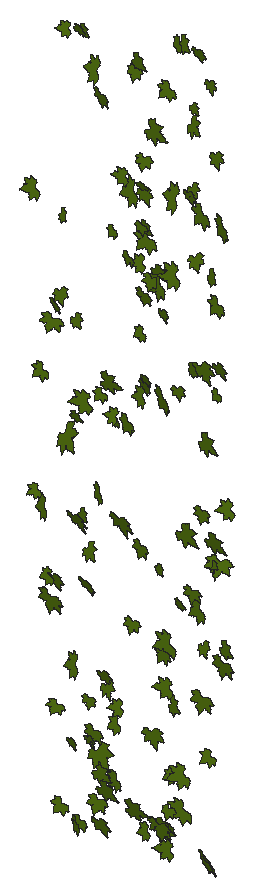
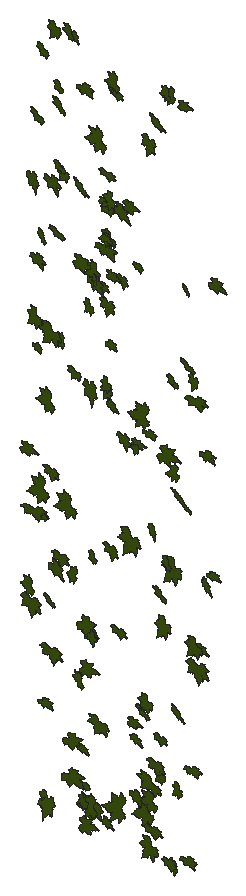
# SketchUp Ruby script. Lengths in inches.
U = 1.inch
M = Sketchup.active_model
def pt(a) = Geom::Point3d.new(a.map { |v| v * U })
def face(e, loops, mat)
  f = e.add_face(loops[0].map { |a| pt(a) })
  loops[1..].each { |l| e.add_face(l.map { |a| pt(a) }).erase! }
  f.material = f.back_material = mat if mat
  f
end
# faces: each face lists its corners as indices into pts; further lists are holes
def faces(e, pts, list, mat = nil) = list.each { |f| face(e, (f[0].is_a?(Array) ? f : [f]).map { |l| l.map { |i| pts[i] } }, mat) }
# xy, xz, yz: faces in a plane at the given z, y or x. An outline is a flat list of corners, or four numbers for a rectangle; further outlines are holes
def ring(l) = l.size == 4 ? [[l[0], l[1]], [l[2], l[1]], [l[2], l[3]], [l[0], l[3]]] : l.each_slice(2).to_a
def flat(e, list, mat, &to3) = list.each { |f| face(e, (f[0].is_a?(Array) ? f : [f]).map { |l| ring(l).map { |u, v| to3.(u, v) } }, mat) }
def xy(e, z, list, mat = nil) = flat(e, list, mat) { |x, y| [x, y, z] }
def xz(e, y, list, mat = nil) = flat(e, list, mat) { |x, z| [x, y, z] }
def yz(e, x, list, mat = nil) = flat(e, list, mat) { |y, z| [x, y, z] }
def lines(e, pts, list) = list.each { |a, b| e.add_line(pt(pts[a]), pt(pts[b])) }
# prism: a flat outline (further loops are holes) pulled along v
def prism(e, loops, v, mat = nil)
  f = face(e, loops, mat); d = Geom::Vector3d.new(v.map { |x| x * U })
  f.pushpull(f.normal.samedirection?(d) ? d.length : -d.length)
end
def box(e, o, s, mat = nil) = prism(e, [[o, [o[0] + s[0], o[1], o[2]], [o[0] + s[0], o[1] + s[1], o[2]], [o[0], o[1] + s[1], o[2]]]], [0, 0, s[2]], mat)
def at(x, y, z, deg = 0) = Geom::Transformation.translation(pt([x, y, z])) * Geom::Transformation.rotation(ORIGIN, Z_AXIS, deg.degrees)
def axes(o, x, y, z) = Geom::Transformation.new([*x, 0, *y, 0, *z, 0, *pt(o).to_a, 1])
def part(name) = M.definitions.add(name)
# library, detail: a bought-in or finely detailed component or shape, given as its bounding box
def library(name, o, s) = part(name).tap { |d| box(d.entities, o, s) }
def detail(e, o, s) = box(e.add_group.entities, o, s)
def put(e, d, t, mat = nil) = e.add_instance(d, t).tap { |i| i.material = mat if mat }
def group(e, t, mat = nil) = e.add_group.tap { |g| g.transformation = t; g.material = mat if mat }.entities
root = M.entities
M.materials.add("[Vegetation Blur 03]").color = [83, 114, 18]
c1 = part("ivy")
xy(c1.entities,0,[[0.782,0,0.786,0,0.787,0.005,0.789,0.009,0.821,0.072,0.875,0.147,1.001,0.272,1.073,0.331,1.137,0.363,1.178,0.379,1.223,0.384,1.272,0.383,1.311,0.374,1.36,0.355,1.399,0.334,1.491,0.285,1.541,0.244,1.583,0.199,1.617,0.15,1.64,0.128,1.662,0.115,1.717,0.105,1.745,0.093,1.784,0.054,1.819,0.057,1.854,0.064,1.882,0.075,1.896,0.074,1.91,0.071,1.937,0.063,1.964,0.053,1.99,0.038,2.016,0.015,2.034,0.002,2.04,0,2.038,0.003,2.036,0.007,2.033,0.038,2.036,0.068,2.045,0.1,2.055,0.116,2.064,0.123,2.077,0.129,2.088,0.129,2.106,0.132,2.118,0.13,2.179,0.132,2.207,0.133,2.225,0.133,2.242,0.138,2.22,0.162,2.207,0.186,2.206,0.213,2.212,0.236,2.228,0.262,2.247,0.274,2.298,0.283,2.355,0.294,2.37,0.296,2.376,0.295,2.377,0.3,2.377,0.303,2.385,0.329,2.411,0.37,2.426,0.392,2.449,0.407,2.511,0.426,2.561,0.444,2.619,0.466,2.589,0.469,2.561,0.476,2.501,0.5,2.449,0.516,2.424,0.523,2.401,0.535,2.377,0.556,2.372,0.568,2.36,0.575,2.268,0.586,2.225,0.592,2.207,0.599,2.194,0.61,2.143,0.65,2.13,0.664,2.122,0.682,2.123,0.7,2.13,0.719,2.148,0.75,2.17,0.781,2.195,0.807,2.221,0.828,2.284,0.874,2.291,0.88,2.288,0.887,2.276,0.9,2.267,0.916,2.265,0.933,2.273,0.967,2.292,1.002,2.313,1.03,2.334,1.054,2.348,1.067,2.358,1.074,2.363,1.076,2.362,1.081,2.35,1.094,2.347,1.11,2.35,1.143,2.359,1.18,2.385,1.254,2.415,1.324,2.448,1.393,2.45,1.4,2.446,1.398,2.44,1.394,2.427,1.383,2.402,1.36,2.376,1.339,2.345,1.324,2.305,1.309,2.282,1.303,2.273,1.306,2.245,1.294,2.212,1.287,2.187,1.291,2.163,1.301,2.142,1.316,2.134,1.327,2.124,1.325,2.09,1.292,2.053,1.259,2.014,1.234,1.973,1.215,1.954,1.21,1.931,1.208,1.909,1.212,1.893,1.22,1.879,1.233,1.872,1.248,1.867,1.281,1.864,1.319,1.821,1.258,1.773,1.197,1.726,1.141,1.698,1.121,1.679,1.116,1.666,1.117,1.647,1.122,1.632,1.129,1.62,1.141,1.617,1.154,1.617,1.219,1.621,1.254,1.623,1.268,1.623,1.281,1.618,1.314,1.606,1.346,1.603,1.375,1.607,1.403,1.603,1.467,1.599,1.499,1.605,1.525,1.614,1.552,1.629,1.577,1.635,1.589,1.629,1.587,1.618,1.582,1.596,1.566,1.581,1.556,1.568,1.552,1.557,1.55,1.545,1.553,1.531,1.562,1.522,1.572,1.504,1.591,1.486,1.611,1.474,1.631,1.457,1.666,1.455,1.684,1.457,1.698,1.452,1.715,1.444,1.728,1.424,1.754,1.419,1.772,1.423,1.786,1.434,1.819,1.444,1.848,1.446,1.855,1.44,1.861,1.43,1.867,1.386,1.904,1.349,1.948,1.326,1.973,1.31,1.995,1.288,2.048,1.284,2.153,1.287,2.254,1.284,2.255,1.282,2.253,1.278,2.247,1.274,2.237,1.266,2.216,1.226,2.125,1.208,2.076,1.184,2.033,1.155,1.984,1.135,1.942,1.111,1.899,1.083,1.861,1.053,1.85,1.059,1.83,1.061,1.809,1.056,1.79,1.049,1.767,1.04,1.749,1.018,1.733,0.994,1.726,0.942,1.734,0.95,1.6875,0.944,1.645,0.932,1.608,0.911,1.585,0.881,1.58,0.854,1.582,0.828,1.588,0.785,1.618,0.773,1.625,0.775,1.614,0.779,1.598,0.796,1.502,0.818,1.402,0.861,1.283,0.882,1.224,0.894,1.174,0.892,1.148,0.886,1.123,0.881,1.107,0.872,1.099,0.849,1.094,0.818,1.092,0.789,1.098,0.762,1.107,0.753,1.113,0.721,1.139,0.698,1.163,0.678,1.194,0.665,1.224,0.628,1.28,0.612,1.312,0.606,1.327,0.606,1.314,0.599,1.282,0.594,1.267,0.581,1.256,0.544,1.245,0.512,1.244,0.473,1.249,0.444,1.256,0.382,1.288,0.339,1.306,0.324,1.316,0.317,1.324,0.309,1.326,0.27,1.314,0.227,1.313,0.185,1.3125,0.152,1.317,0.122,1.328,0.092,1.345,0.073,1.353,0.079,1.338,0.092,1.308,0.117,1.249,0.13,1.215,0.139,1.164,0.147,1.148,0.157,1.136,0.163,1.122,0.174,1.086,0.177,1.067,0.182,1.054,0.186,1.043,0.191,1.038,0.211,1.028,0.237,1.005,0.25,0.974,0.253,0.96,0.25,0.944,0.242,0.914,0.243,0.906,0.249,0.902,0.26,0.894,0.289,0.88,0.307,0.873,0.322,0.862,0.364,0.799,0.403,0.738,0.431,0.709,0.439,0.691,0.441,0.678,0.4375,0.66,0.428,0.645,0.394,0.623,0.303,0.594,0.255,0.581,0.214,0.577,0.179,0.573,0.173,0.568,0.175,0.561,0.167,0.55,0.141,0.523,0.113,0.503,0.077,0.49,0.045,0.486,0.026,0.485,0.019,0.486,0.011,0.483,0,0.471,0.014,0.467,0.044,0.455,0.058,0.447,0.07,0.438,0.097,0.411,0.125,0.394,0.158,0.377,0.174,0.366,0.182,0.359,0.185,0.361,0.242,0.331,0.253,0.316,0.258,0.303,0.262,0.283,0.274,0.278,0.308,0.274,0.341,0.252,0.366,0.226,0.366,0.222,0.37,0.22,0.38,0.221,0.395,0.221,0.425,0.216,0.45,0.207,0.465,0.192,0.473,0.178,0.484,0.15,0.489,0.116,0.483,0.089,0.468,0.058,0.45,0.035,0.435,0.018,0.429,0.011,0.434,0.012,0.438,0.014,0.469,0.019,0.542,0.016,0.581,0.015,0.612,0.027,0.68,0.055,0.696,0.057,0.712,0.052,0.73,0.045,0.741,0.036,0.766,0.014]])
put(root,c1,axes([10.7,173.7,38.86],[0.22705,-0.11945,-0.35491],[-0.43835,-0.02,-0.18572],[-0.01818,-1.0093,0.04569]),"[Vegetation Blur 03]")
put(root,c1,axes([10.72,173.7,22.84],[0.22258,-0.06561,-0.19839],[-0.24493,-0.08915,-0.17839],[0.01076,-0.67235,0.04301]),"[Vegetation Blur 03]")
put(root,c1,axes([10.9375,173.7,29.33],[0.3254,-0.08509,-0.21734],[-0.269,-0.05049,-0.26515],[-0.01633,-0.86378,0.03691]),"[Vegetation Blur 03]")
put(root,c1,axes([11.23,173.7,22.41],[0.27571,-0.25978,-0.33675],[-0.40528,0.18997,-0.24407],[-0.14812,-1.00337,0.04098]),"[Vegetation Blur 03]")
put(root,c1,axes([11.59,173.7,18.67],[0.1748,-0.10036,-0.26156],[-0.32362,-0.01023,-0.14344],[-0.01895,-0.75115,0.0369]),"[Vegetation Blur 03]")
put(root,c1,axes([11.22,173.7,32.02],[0.48108,0.0091,-0.09014],[-0.10924,-0.11608,-0.39016],[0.0169,-1.00907,0.04407]),"[Vegetation Blur 03]")
put(root,c1,axes([10.97,173.7,17.55],[0.65346,-0.15996,-0.07236],[-0.08578,0.05992,-0.53686],[-0.0809,-1.3557,-0.01519]),"[Vegetation Blur 03]")
put(root,c1,axes([11.625,173.7,11.875],[0.36198,-0.00364,-0.10329],[-0.12566,-0.10485,-0.29275],[0.01516,-0.7821,0.03972]),"[Vegetation Blur 03]")
put(root,c1,axes([11.57,173.7,32.88],[0.3582,-0.18702,-0.03708],[-0.03384,0.10347,-0.29982],[-0.09581,-0.73577,-0.03274]),"[Vegetation Blur 03]")
put(root,c1,axes([11.21,173.7,18.26],[0.44883,-0.14962,0.17944],[0.22549,0.05754,-0.36812],[-0.05276,-1.02686,-0.04677]),"[Vegetation Blur 03]")
put(root,c1,axes([11.97,173.7,6.9],[0.37574,-0.07096,-0.15978],[-0.19839,-0.07956,-0.3052],[-0.01253,-0.86822,0.04103]),"[Vegetation Blur 03]")
put(root,c1,axes([11.74,173.7,33.23],[0.32579,-0.0019,0.20222],[0.24053,-0.19974,-0.25841],[-0.05947,-0.81825,0.06261]),"[Vegetation Blur 03]")
put(root,c1,axes([12.07,173.7,37.17],[0.07732,0.04701,0.24249],[0.28519,-0.19481,-0.05463],[-0.0864,-0.60099,0.03668]),"[Vegetation Blur 03]")
put(root,c1,axes([12.75,173.7,47.72],[0.09099,-0.0894,-0.27257],[-0.33609,-0.07013,-0.07111],[0.02177,-0.70885,0.04141]),"[Vegetation Blur 03]")
put(root,c1,axes([11.88,173.7,25.39],[0.26041,0.16269,0.49935],[0.59768,-0.40532,-0.18684],[-0.15294,-1.30696,0.1201]),"[Vegetation Blur 03]")
put(root,c1,axes([13.15,173.7,14.82],[0.25932,-0.29593,-0.35358],[-0.43934,0.11655,-0.22996],[-0.12392,-1.03246,0.07539]),"[Vegetation Blur 03]")
put(root,c1,axes([12.51,173.7,10.03],[0.27088,-0.15261,0.15464],[0.19269,-0.01614,-0.22733],[-0.06536,-0.68006,-0.0293]),"[Vegetation Blur 03]")
put(root,c1,axes([12.92,173.7,6.22],[0.37274,-0.27698,-0.10257],[-0.11734,0.09274,-0.32343],[-0.14192,-0.80413,-0.00197]),"[Vegetation Blur 03]")
put(root,c1,axes([12.75,173.7,26.97],[0.1451,-0.1312,0.25798],[0.3214,0.00081,-0.12034],[-0.02623,-0.71573,-0.04743]),"[Vegetation Blur 03]")
put(root,c1,axes([12.72,173.7,32.03],[0.20968,0.01131,0.23173],[0.28004,-0.12895,-0.16779],[-0.0472,-0.71481,0.03394]),"[Vegetation Blur 03]")
put(root,c1,axes([13.78,173.7,28.72],[0.17219,-0.03701,-0.43547],[-0.53302,-0.07752,-0.13935],[0.03036,-1.15115,0.02338]),"[Vegetation Blur 03]")
put(root,c1,axes([13.04,173.7,6.29],[0.37414,-0.10141,-0.07585],[-0.09511,-0.0243,-0.3074],[-0.04493,-0.79294,0.01912]),"[Vegetation Blur 03]")
put(root,c1,axes([12.45,173.7,21.96],[0.55336,-0.2755,0.17895],[0.23761,0.14136,-0.45516],[-0.0977,-1.21665,-0.0934]),"[Vegetation Blur 03]")
put(root,c1,axes([12.97,173.7,47.37],[0.16816,-0.15089,0.24654],[0.3088,-0.00002,-0.1403],[-0.03567,-0.71145,-0.05229]),"[Vegetation Blur 03]")
put(root,c1,axes([13.19,173.7,21.9],[0.13772,-0.02232,0.26418],[0.31478,-0.16115,-0.11144],[-0.07624,-0.70573,0.01709]),"[Vegetation Blur 03]")
put(root,c1,axes([13.25,173.7,47.37],[0.14289,-0.07488,0.25812],[0.31299,-0.09737,-0.11985],[-0.0582,-0.70749,-0.01082]),"[Vegetation Blur 03]")
put(root,c1,axes([13.14,173.7,18.76],[0.46892,-0.24319,0.11777],[0.16224,0.13537,-0.38629],[-0.09203,-1.00049,-0.08089]),"[Vegetation Blur 03]")
put(root,c1,axes([13.48,173.7,12.71],[0.35341,-0.05372,0.02619],[0.03014,-0.05475,-0.28854],[-0.02834,-0.72817,0.01976]),"[Vegetation Blur 03]")
put(root,c1,axes([13.51,173.7,10.5],[0.29444,-0.13699,0.14225],[0.1786,0.0132,-0.24425],[-0.05394,-0.70397,-0.03226]),"[Vegetation Blur 03]")
put(root,c1,axes([13.42,173.7,20.09],[0.20883,0.04815,0.31421],[0.37772,-0.20796,-0.1622],[-0.0781,-0.87697,0.05572]),"[Vegetation Blur 03]")
put(root,c1,axes([14.55,173.7,46.43],[0.1383,-0.27518,-0.42018],[-0.52123,0.14835,-0.12955],[-0.10615,-1.08693,0.0887]),"[Vegetation Blur 03]")
put(root,c1,axes([13.69,173.7,11.3],[0.4987,-0.12613,-0.04723],[-0.0598,-0.02572,-0.40975],[-0.05942,-1.03278,0.01597]),"[Vegetation Blur 03]")
put(root,c1,axes([14.34,173.7,24.12],[0.31941,-0.24553,-0.21108],[-0.24847,0.1507,-0.27802],[-0.13923,-0.8322,0.01193]),"[Vegetation Blur 03]")
put(root,c1,axes([13.91,173.7,7.7],[0.48615,-0.06506,-0.03255],[-0.04363,-0.12709,-0.39413],[-0.0262,-0.99568,0.05243]),"[Vegetation Blur 03]")
put(root,c1,axes([14.4,173.7,29.18],[0.29981,-0.06525,-0.13535],[-0.1686,-0.07812,-0.24283],[-0.00912,-0.70071,0.03968]),"[Vegetation Blur 03]")
put(root,c1,axes([14.13,173.7,44.84],[0.50217,-0.23211,-0.02067],[-0.01614,0.08923,-0.41886],[-0.11447,-1.03084,-0.03161]),"[Vegetation Blur 03]")
put(root,c1,axes([13.66,173.7,9.65],[0.43574,0.04341,0.40329],[0.4922,-0.17124,-0.35133],[-0.04861,-1.34487,0.05775]),"[Vegetation Blur 03]")
put(root,c1,axes([13.98,173.7,8.53],[0.18345,-0.01602,0.41607],[0.50825,-0.08298,-0.14976],[-0.04057,-1.11184,0.00518]),"[Vegetation Blur 03]")
put(root,c1,axes([13.875,173.7,6.36],[0.49317,-0.18476,0.20262],[0.2548,0.0498,-0.40595],[-0.06909,-1.1351,-0.05079]),"[Vegetation Blur 03]")
put(root,c1,axes([14.24,173.7,14.15],[0.36419,-0.14328,0.1768],[0.2225,0.04791,-0.29916],[-0.04769,-0.87068,-0.04556]),"[Vegetation Blur 03]")
put(root,c1,axes([14.2,173.7,7.85],[0.29611,-0.16504,0.41768],[0.51687,0.01316,-0.24325],[-0.03458,-1.21665,-0.05929]),"[Vegetation Blur 03]")
put(root,c1,axes([14.48,173.7,13.44],[0.29238,-0.00543,0.2431],[0.28843,-0.20948,-0.23179],[-0.07444,-0.83296,0.05671]),"[Vegetation Blur 03]")
put(root,c1,axes([15.62,173.7,28.375],[0.04403,-0.12753,-0.27738],[-0.34532,-0.03734,-0.03381],[0.01033,-0.70424,0.05202]),"[Vegetation Blur 03]")
put(root,c1,axes([15.09,173.7,37.94],[0.27643,-0.11245,-0.0959],[-0.1208,-0.01738,-0.22873],[-0.04691,-0.61786,0.02389]),"[Vegetation Blur 03]")
put(root,c1,axes([14.59,173.7,29.11],[0.08822,-0.12322,0.46198],[0.56917,0.00464,-0.0722],[-0.00698,-1.17889,-0.04857]),"[Vegetation Blur 03]")
put(root,c1,axes([15.27,173.7,9.4],[0.34978,-0.17504,-0.23097],[-0.28247,0.06704,-0.29293],[-0.08681,-0.92345,0.02252]),"[Vegetation Blur 03]")
put(root,c1,axes([15.43,173.7,12.375],[0.28202,-0.18926,-0.22565],[-0.28437,-0.00619,-0.23592],[-0.06351,-0.81269,0.05435]),"[Vegetation Blur 03]")
put(root,c1,axes([15.18,173.7,27.98],[0.28723,-0.15203,-0.02555],[-0.02588,0.0511,-0.24162],[-0.07595,-0.59236,-0.01429]),"[Vegetation Blur 03]")
put(root,c1,axes([15.79,173.7,13.22],[0.11929,-0.10597,-0.2818],[-0.34889,-0.06251,-0.09467],[0.01224,-0.74914,0.04776]),"[Vegetation Blur 03]")
put(root,c1,axes([16.11,173.7,41.16],[0.05825,-0.05857,-0.32384],[-0.39732,-0.0501,-0.04618],[0.02002,-0.82377,0.02584]),"[Vegetation Blur 03]")
put(root,c1,axes([14.96,173.7,22.8],[0.63866,-0.23189,0.12864],[0.16822,0.10928,-0.52532],[-0.09614,-1.34925,-0.06466]),"[Vegetation Blur 03]")
put(root,c1,axes([15.83,173.7,28.36],[0.44792,-0.20906,-0.13241],[-0.16237,0.03502,-0.37455],[-0.10139,-0.9797,0.01487]),"[Vegetation Blur 03]")
put(root,c1,axes([15.92,173.7,36.87],[0.35103,-0.1488,-0.07514],[-0.0909,0.03087,-0.29249],[-0.07377,-0.74614,0.00288]),"[Vegetation Blur 03]")
put(root,c1,axes([16.41,173.7,40.93],[0.36429,-0.26691,-0.39719],[-0.49048,0.09297,-0.30946],[-0.1145,-1.24751,0.06192]),"[Vegetation Blur 03]")
put(root,c1,axes([16,173.7,17.7],[0.40879,-0.06868,-0.00639],[-0.01176,-0.09983,-0.33231],[-0.0322,-0.83542,0.04024]),"[Vegetation Blur 03]")
put(root,c1,axes([16.21,173.7,46.72],[0.38042,-0.08348,0.02066],[0.01844,-0.12918,-0.30833],[-0.04412,-0.77385,0.04924]),"[Vegetation Blur 03]")
put(root,c1,axes([17.07,173.7,37.02],[0.14335,-0.13764,-0.29117],[-0.36286,-0.03379,-0.11648],[-0.00945,-0.79049,0.05568]),"[Vegetation Blur 03]")
put(root,c1,axes([17.05,173.7,30.09],[0.18991,-0.19032,-0.31472],[-0.38839,0.08836,-0.16451],[-0.08006,-0.88012,0.05154]),"[Vegetation Blur 03]")
put(root,c1,axes([16.05,173.7,7.26],[0.11966,-0.19885,0.48664],[0.60405,0.04067,-0.09632],[0.00062,-1.25082,-0.0805]),"[Vegetation Blur 03]")
put(root,c1,axes([16.91,173.7,33.25],[0.22039,-0.10268,-0.20891],[-0.2592,-0.01,-0.18136],[-0.02883,-0.69502,0.03347]),"[Vegetation Blur 03]")
put(root,c1,axes([16.34,173.7,46.71],[0.15082,-0.08194,0.36497],[0.44384,-0.11913,-0.12637],[-0.06768,-0.96384,-0.01541]),"[Vegetation Blur 03]")
put(root,c1,axes([16.52,173.7,21.99],[0.46442,-0.17928,-0.04706],[-0.05947,-0.00913,-0.38545],[-0.0859,-0.96299,0.01241]),"[Vegetation Blur 03]")
put(root,c1,axes([16.53,173.7,38.55],[0.32611,-0.0735,0.11387],[0.13621,-0.07341,-0.2673],[-0.04678,-0.72621,0.01549]),"[Vegetation Blur 03]")
put(root,c1,axes([17.24,173.7,7.31],[0.2031,-0.14404,-0.26055],[-0.32267,0.0347,-0.17055],[-0.052,-0.77785,0.04064]),"[Vegetation Blur 03]")
put(root,c1,axes([16.54,173.7,40.54],[0.28631,-0.17737,0.19402],[0.25002,0.08801,-0.2331],[-0.03783,-0.76071,-0.07221]),"[Vegetation Blur 03]")
put(root,c1,axes([16.63,173.7,35.22],[0.46399,-0.15608,-0.0301],[-0.03246,0.06122,-0.3832],[-0.07784,-0.95586,-0.01963]),"[Vegetation Blur 03]")
put(root,c1,axes([16.68,173.7,42.21],[0.40348,-0.0468,0.02113],[0.02171,-0.14086,-0.32526],[-0.02676,-0.81998,0.05467]),"[Vegetation Blur 03]")
put(root,c1,axes([16.96,173.7,38.51],[0.49046,-0.12487,-0.25125],[-0.31171,-0.05916,-0.40067],[-0.03597,-1.19015,0.04628]),"[Vegetation Blur 03]")
put(root,c1,axes([16.73,173.7,30.4],[0.3929,-0.21833,0.06927],[0.09371,0.04854,-0.33],[-0.09838,-0.82573,-0.03771]),"[Vegetation Blur 03]")
put(root,c1,axes([16.59,173.7,40.21],[0.36838,-0.06003,0.20905],[0.25298,-0.09287,-0.30112],[-0.04965,-0.91861,0.01678]),"[Vegetation Blur 03]")
put(root,c1,axes([16.8125,173.7,30.58],[0.28308,-0.16005,0.12566],[0.16212,0.03888,-0.23548],[-0.05892,-0.66197,-0.04421]),"[Vegetation Blur 03]")
put(root,c1,axes([16.75,173.7,38.23],[0.16779,-0.0883,0.30239],[0.37001,-0.06611,-0.13979],[-0.04708,-0.83437,-0.02093]),"[Vegetation Blur 03]")
put(root,c1,axes([17.1,173.7,36.12],[0.43256,-0.06671,-0.01604],[-0.02325,-0.10108,-0.35159],[-0.02994,-0.88528,0.04135]),"[Vegetation Blur 03]")
put(root,c1,axes([16.89,173.7,12.09],[0.51003,-0.05161,0.17077],[0.20792,-0.06034,-0.4165],[-0.03431,-1.13281,0.01441]),"[Vegetation Blur 03]")
put(root,c1,axes([17.82,173.7,36.52],[0.43677,-0.25618,-0.34823],[-0.42807,0.08886,-0.36791],[-0.11962,-1.25334,0.04509]),"[Vegetation Blur 03]")
put(root,c1,axes([17.07,173.7,43.19],[0.18628,-0.03587,0.49266],[0.60208,-0.08964,-0.15266],[-0.04677,-1.29689,-0.00307]),"[Vegetation Blur 03]")
put(root,c1,axes([17.43,173.7,36.26],[0.26264,-0.10696,0.28896],[0.35555,-0.0243,-0.21667],[-0.0405,-0.90682,-0.02828]),"[Vegetation Blur 03]")
put(root,c1,axes([17.3,173.7,7.66],[0.62439,-0.15847,0.04406],[0.05688,0.04229,-0.51297],[-0.0749,-1.28898,-0.02225]),"[Vegetation Blur 03]")
put(root,c1,axes([17.6875,173.7,20.77],[0.18692,-0.08145,0.20202],[0.24238,-0.1034,-0.15594],[-0.06396,-0.62987,-0.00053]),"[Vegetation Blur 03]")
put(root,c1,axes([17.81,173.7,30.54],[0.55558,-0.31709,-0.23093],[-0.26347,0.22092,-0.46992],[-0.18545,-1.26384,-0.0242]),"[Vegetation Blur 03]")
put(root,c1,axes([18.65,173.7,15.32],[0.10909,-0.05884,-0.38294],[-0.46937,-0.06819,-0.08742],[0.02587,-0.98895,0.02881]),"[Vegetation Blur 03]")
put(root,c1,axes([18.73,173.7,6.81],[0.07011,-0.04175,-0.39035],[-0.47768,-0.07166,-0.05594],[0.03155,-0.99215,0.02047]),"[Vegetation Blur 03]")
put(root,c1,axes([17.91,173.7,17.06],[0.4568,-0.18649,-0.14633],[-0.18134,0.01163,-0.3794],[-0.08646,-1.00976,0.02265]),"[Vegetation Blur 03]")
put(root,c1,axes([18.45,173.7,17.83],[0.34831,-0.13161,-0.42418],[-0.52189,0.01831,-0.28634],[-0.04303,-1.28736,0.03929]),"[Vegetation Blur 03]")
put(root,c1,axes([17.86,173.7,34.4],[0.29752,-0.1463,0.14185],[0.17418,-0.03541,-0.24908],[-0.07018,-0.70816,-0.01685]),"[Vegetation Blur 03]")
put(root,c1,axes([17.7,173.7,6.9],[0.12855,-0.09811,0.43066],[0.52964,-0.00555,-0.1055],[-0.01392,-1.1176,-0.03728]),"[Vegetation Blur 03]")
put(root,c1,axes([18.3,173.7,46.65],[0.37323,-0.08724,-0.21133],[-0.2619,-0.06711,-0.30372],[-0.01607,-0.93236,0.04164]),"[Vegetation Blur 03]")
put(root,c1,axes([18.65,173.7,10.68],[0.22279,-0.12525,-0.19809],[-0.24846,-0.03124,-0.18302],[-0.02974,-0.67725,0.04508]),"[Vegetation Blur 03]")
put(root,c1,axes([18.24,173.7,8.61],[0.33968,-0.06301,-0.00772],[-0.01455,-0.11855,-0.2742],[-0.02856,-0.68915,0.04788]),"[Vegetation Blur 03]")
put(root,c1,axes([18.99,173.7,37.27],[0.22309,-0.1604,-0.43567],[-0.53899,-0.01598,-0.18291],[-0.02282,-1.19045,0.06116]),"[Vegetation Blur 03]")
put(root,c1,axes([19.18,173.7,41.38],[0.14321,-0.30149,-0.44399],[-0.54717,0.20081,-0.13901],[-0.13425,-1.14006,0.09293]),"[Vegetation Blur 03]")
put(root,c1,axes([18.2,173.7,7.37],[0.20518,-0.11933,0.20995],[0.26085,-0.0065,-0.17038],[-0.03866,-0.67709,-0.03537]),"[Vegetation Blur 03]")
put(root,c1,axes([18.49,173.7,13.59],[0.06873,0.01711,0.34805],[0.41669,-0.19262,-0.05332],[-0.09114,-0.86777,0.0187]),"[Vegetation Blur 03]")
put(root,c1,axes([19.0625,173.7,49.22],[0.22954,-0.17233,-0.19599],[-0.23774,0.09106,-0.19805],[-0.09034,-0.67751,0.02323]),"[Vegetation Blur 03]")
put(root,c1,axes([19.09,173.7,9.28],[0.4097,-0.04709,-0.34938],[-0.42867,-0.05903,-0.33358],[0.00494,-1.21793,0.02968]),"[Vegetation Blur 03]")
put(root,c1,axes([19.29,173.7,11.16],[0.31711,-0.08877,-0.37028],[-0.45541,-0.10498,-0.25583],[0.01733,-1.13422,0.05266]),"[Vegetation Blur 03]")
put(root,c1,axes([18.63,173.7,30.63],[0.33984,-0.05336,0.11192],[0.13528,-0.05673,-0.27786],[-0.03432,-0.75199,0.01302]),"[Vegetation Blur 03]")
put(root,c1,axes([18.99,173.7,19.22],[0.06463,-0.12992,0.26421],[0.32679,-0.06667,-0.0584],[-0.04465,-0.67604,-0.04502]),"[Vegetation Blur 03]")
put(root,c1,axes([19.0625,173.7,48.58],[0.1212,0.00874,0.32904],[0.39357,-0.19062,-0.09576],[-0.08752,-0.84508,0.025]),"[Vegetation Blur 03]")
put(root,c1,axes([18.82,173.7,22.82],[0.30964,-0.0676,0.45983],[0.56279,-0.06237,-0.25387],[-0.0424,-1.3215,-0.01154]),"[Vegetation Blur 03]")
put(root,c1,axes([19.34,173.7,41.17],[0.34101,-0.13421,0.11002],[0.1371,0.00224,-0.28262],[-0.06025,-0.75456,-0.02041]),"[Vegetation Blur 03]")
put(root,c1,axes([19.43,173.7,20.53],[0.44619,-0.06474,-0.00167],[-0.00306,-0.02944,-0.36486],[-0.03138,-0.91771,0.01182]),"[Vegetation Blur 03]")
put(root,c1,axes([19.68,173.7,31.7],[0.0683,-0.05119,0.27634],[0.33407,-0.11649,-0.05839],[-0.06049,-0.70118,-0.01047]),"[Vegetation Blur 03]")
put(root,c1,axes([19.57,173.7,41.29],[0.21707,0.00977,0.22202],[0.26718,-0.14285,-0.17301],[-0.05136,-0.70178,0.03831]),"[Vegetation Blur 03]")
put(root,c1,axes([19.55,173.7,44.37],[0.13518,0.07282,0.36034],[0.43243,-0.22734,-0.10083],[-0.09589,-0.9226,0.05329]),"[Vegetation Blur 03]")
put(root,c1,axes([19.71,173.7,45.61],[0.18338,-0.0476,0.19783],[0.23906,-0.08339,-0.15076],[-0.04624,-0.61987,0.00509]),"[Vegetation Blur 03]")
put(root,c1,axes([20.21,173.7,20.17],[0.36665,-0.19895,-0.32997],[-0.4044,0.08632,-0.30749],[-0.09631,-1.11984,0.03492]),"[Vegetation Blur 03]")
put(root,c1,axes([19.61,173.7,37.73],[0.33502,0.02499,0.20079],[0.2423,-0.1873,-0.26561],[-0.04435,-0.83458,0.06562]),"[Vegetation Blur 03]")
put(root,c1,axes([19.81,173.7,48.86],[0.38814,-0.14356,0.10109],[0.12917,0.04667,-0.31993],[-0.05936,-0.83711,-0.03517]),"[Vegetation Blur 03]")
put(root,c1,axes([20.19,173.7,40.94],[0.49987,-0.22483,-0.22694],[-0.27931,0.04426,-0.41667],[-0.10606,-1.17624,0.0277]),"[Vegetation Blur 03]")
put(root,c1,axes([19.91,173.7,15.29],[0.58789,-0.11281,-0.04556],[-0.05859,-0.05769,-0.48112],[-0.05185,-1.21383,0.0271]),"[Vegetation Blur 03]")
put(root,c1,axes([20.05,173.7,24.92],[0.43658,-0.10423,0.00392],[0.00224,-0.04583,-0.35826],[-0.05083,-0.89729,0.01784]),"[Vegetation Blur 03]")
put(root,c1,axes([19.74,173.7,32.21],[0.52256,-0.08904,0.24501],[0.30058,-0.01277,-0.42774],[-0.04062,-1.24009,-0.01319]),"[Vegetation Blur 03]")
put(root,c1,axes([20.21,173.7,17.52],[0.23663,-0.00308,0.21961],[0.25991,-0.18831,-0.18695],[-0.06967,-0.71292,0.04843]),"[Vegetation Blur 03]")
put(root,c1,axes([20.81,173.7,12.46],[0.296,-0.08214,-0.20649],[-0.25613,-0.08908,-0.23898],[-0.00188,-0.79632,0.04803]),"[Vegetation Blur 03]")
put(root,c1,axes([20.36,173.7,6.66],[0.4103,-0.202,-0.00421],[0.00893,0.12198,-0.34084],[-0.09789,-0.83552,-0.04874]),"[Vegetation Blur 03]")
put(root,c1,axes([20.2,173.7,7.04],[0.61856,-0.3329,-0.06965],[-0.05285,0.26763,-0.51381],[-0.1751,-1.25675,-0.09097]),"[Vegetation Blur 03]")
put(root,c1,axes([20.21,173.7,27.99],[0.19561,-0.07372,0.44835],[0.54629,-0.12238,-0.16192],[-0.06809,-1.19373,-0.01109]),"[Vegetation Blur 03]")
put(root,c1,axes([20.6,173.7,47.36],[0.32177,-0.10077,0.13804],[0.16444,-0.08743,-0.26534],[-0.06299,-0.74292,0.0125]),"[Vegetation Blur 03]")
put(root,c1,axes([20.72,173.7,22.22],[0.28684,-0.06236,0.1063],[0.12625,-0.08285,-0.23456],[-0.04409,-0.64295,0.01992]),"[Vegetation Blur 03]")
put(root,c1,axes([20.78,173.7,36.93],[0.07908,0.01608,0.29029],[0.3424,-0.20709,-0.06032],[-0.09663,-0.72064,0.02381]),"[Vegetation Blur 03]")
put(root,c1,axes([21.25,173.7,31.49],[0.2496,-0.10992,-0.13236],[-0.16418,0.00788,-0.20725],[-0.04691,-0.61248,0.02109]),"[Vegetation Blur 03]")
put(root,c1,axes([21.12,173.7,36.38],[0.42696,-0.16855,-0.18226],[-0.22665,-0.00186,-0.3534],[-0.07216,-0.99152,0.03164]),"[Vegetation Blur 03]")
put(root,c1,axes([20.81,173.7,22.63],[0.56687,0.06013,-0.01984],[-0.01943,-0.18427,-0.45761],[0.03267,-1.15295,0.0721]),"[Vegetation Blur 03]")
put(root,c1,axes([20.56,173.7,23.1],[0.31154,-0.18802,0.42817],[0.53015,-0.00865,-0.25753],[-0.0503,-1.25557,-0.06234]),"[Vegetation Blur 03]")
put(root,c1,axes([20.875,173.7,43.62],[0.34903,-0.06561,0.18456],[0.21828,-0.15404,-0.28357],[-0.06714,-0.84183,0.0375]),"[Vegetation Blur 03]")
put(root,c1,axes([21.43,173.7,40.71],[0.46455,-0.28541,-0.24702],[-0.29064,0.17394,-0.39567],[-0.16241,-1.12761,0.00149]),"[Vegetation Blur 03]")
put(root,c1,axes([20.99,173.7,32.62],[0.36896,-0.184,0.21842],[0.27276,0.00042,-0.30684],[-0.07226,-0.93795,-0.04299]),"[Vegetation Blur 03]")
put(root,c1,axes([21.13,173.7,17.57],[0.60359,-0.16861,-0.0634],[-0.07511,0.04962,-0.497],[-0.08431,-1.25133,-0.01117]),"[Vegetation Blur 03]")
put(root,c1,axes([22.21,173.7,25.94],[0.1638,-0.10041,-0.33523],[-0.41333,-0.07495,-0.13099],[0.01603,-0.90688,0.04794]),"[Vegetation Blur 03]")
put(root,c1,axes([21.49,173.7,17.66],[0.12722,-0.05638,0.35512],[0.42991,-0.13892,-0.10606],[-0.07252,-0.92248,-0.00573]),"[Vegetation Blur 03]")
